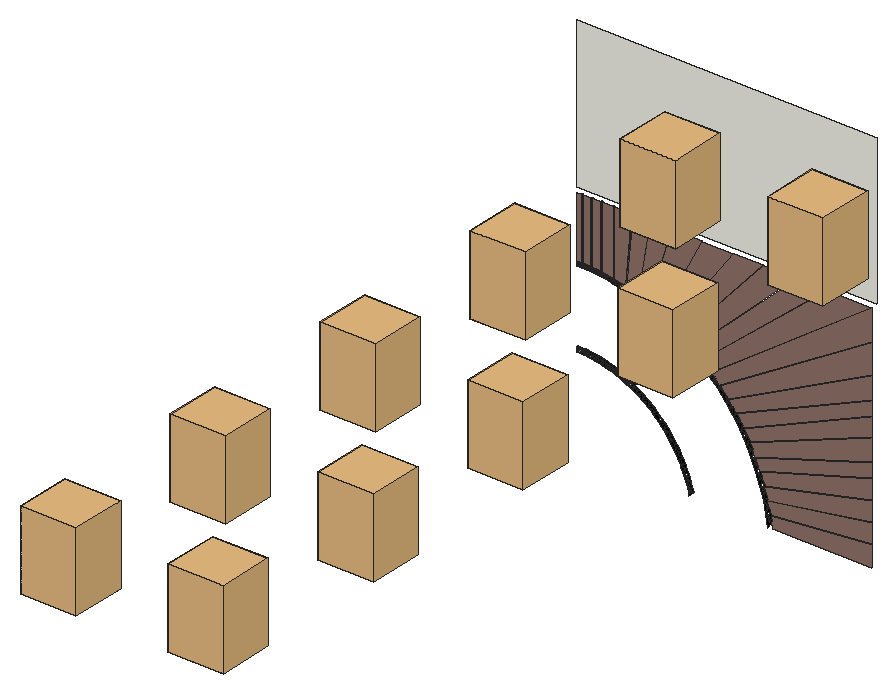
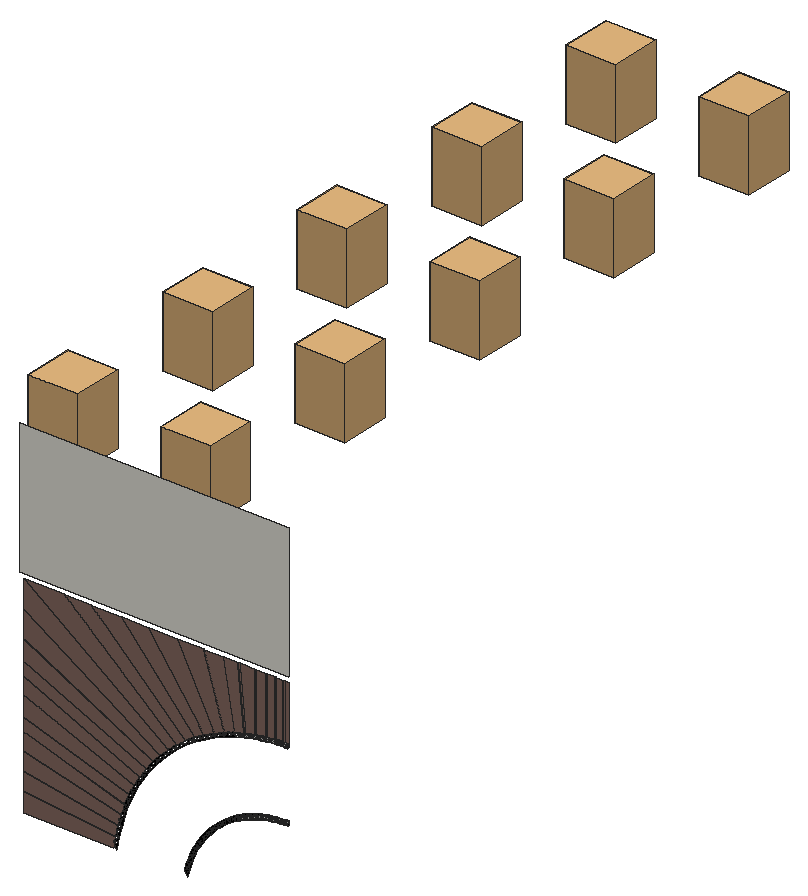
# SketchUp Ruby script. Lengths in inches.
U = 1.inch
M = Sketchup.active_model
def pt(a) = Geom::Point3d.new(a.map { |v| v * U })
def face(e, loops, mat)
  f = e.add_face(loops[0].map { |a| pt(a) })
  loops[1..].each { |l| e.add_face(l.map { |a| pt(a) }).erase! }
  f.material = f.back_material = mat if mat
  f
end
# faces: each face lists its corners as indices into pts; further lists are holes
def faces(e, pts, list, mat = nil) = list.each { |f| face(e, (f[0].is_a?(Array) ? f : [f]).map { |l| l.map { |i| pts[i] } }, mat) }
# xy, xz, yz: faces in a plane at the given z, y or x. An outline is a flat list of corners, or four numbers for a rectangle; further outlines are holes
def ring(l) = l.size == 4 ? [[l[0], l[1]], [l[2], l[1]], [l[2], l[3]], [l[0], l[3]]] : l.each_slice(2).to_a
def flat(e, list, mat, &to3) = list.each { |f| face(e, (f[0].is_a?(Array) ? f : [f]).map { |l| ring(l).map { |u, v| to3.(u, v) } }, mat) }
def xy(e, z, list, mat = nil) = flat(e, list, mat) { |x, y| [x, y, z] }
def xz(e, y, list, mat = nil) = flat(e, list, mat) { |x, z| [x, y, z] }
def yz(e, x, list, mat = nil) = flat(e, list, mat) { |y, z| [x, y, z] }
def lines(e, pts, list) = list.each { |a, b| e.add_line(pt(pts[a]), pt(pts[b])) }
# prism: a flat outline (further loops are holes) pulled along v
def prism(e, loops, v, mat = nil)
  f = face(e, loops, mat); d = Geom::Vector3d.new(v.map { |x| x * U })
  f.pushpull(f.normal.samedirection?(d) ? d.length : -d.length)
end
def box(e, o, s, mat = nil) = prism(e, [[o, [o[0] + s[0], o[1], o[2]], [o[0] + s[0], o[1] + s[1], o[2]], [o[0], o[1] + s[1], o[2]]]], [0, 0, s[2]], mat)
def at(x, y, z, deg = 0) = Geom::Transformation.translation(pt([x, y, z])) * Geom::Transformation.rotation(ORIGIN, Z_AXIS, deg.degrees)
def axes(o, x, y, z) = Geom::Transformation.new([*x, 0, *y, 0, *z, 0, *pt(o).to_a, 1])
def part(name) = M.definitions.add(name)
# library, detail: a bought-in or finely detailed component or shape, given as its bounding box
def library(name, o, s) = part(name).tap { |d| box(d.entities, o, s) }
def detail(e, o, s) = box(e.add_group.entities, o, s)
def put(e, d, t, mat = nil) = e.add_instance(d, t).tap { |i| i.material = mat if mat }
def group(e, t, mat = nil) = e.add_group.tap { |g| g.transformation = t; g.material = mat if mat }.entities
root = M.entities
M.materials.add("Tafisa-Gardenia-or-Gardenia-PM775-4K").color = [246, 245, 235]
M.materials.add("Tafisa-Terrarossa-PM780-4K").color = [148, 117, 107]
M.materials.add("Uniboard-L19-Putty-4K").color = [187, 181, 160]
M.materials.add("[Color M09]").color = [0, 0, 0]
c1 = library("Group\#8",[0,0,0],[8.9,8.9,12.62])
xy(root,78.776,[[101.221,138,101.236,138.157]],"Uniboard-L19-Putty-4K")
xy(root,79.385,[[100.715,138,100.814,138.157],[101.129,138,101.325,138.157]])
xy(root,89.291,[[101.327,138,101.445,138.157],[102.829,138,102.947,138.157],[104.449,138,104.567,138.157],[106.403,138,106.521,138.157],[109.35,138,109.469,138.157]])
xz(root,138,[[100.618,90.118,148.5,114]],"Tafisa-Gardenia-or-Gardenia-PM775-4K")
xz(root,138,[[131.874,51.949,147.791,51.949,147.791,55.307,131.583,53.786,131.719,52.926],[131.564,53.903,147.791,55.426,147.791,58.431,131.159,55.719,131.349,54.869],[131.133,55.835,147.791,58.551,147.791,61.594,130.614,57.622,130.857,56.785],[130.581,57.735,147.791,61.716,147.791,64.758,129.95,59.486,130.245,58.666],[129.91,59.598,147.791,64.881,147.791,67.121,129.171,61.305,129.517,60.506],
  [129.124,61.414,147.791,67.244,147.791,70.662,128.279,63.072,128.675,62.296],[128.226,63.177,147.791,70.788,147.791,73.694,127.279,64.778,127.722,64.029],[127.218,64.881,147.791,73.823,147.791,75.943,126.106,66.518,126.662,65.699],[126.031,66.614,126.059,66.626,147.744,76.051,147.791,76.072,147.791,79.556,124.893,68.082,125.499,67.3],[124.812,68.173,124.84,68.187,147.738,79.662,147.791,79.689,147.791,84.298,123.584,69.566,124.238,68.824],
  [123.498,69.652,123.522,69.667,147.73,84.398,147.791,84.436,147.791,89.291,122.184,70.966],[122.093,71.046,122.116,71.062,147.588,89.291,140.748,89.291,120.7,72.275,121.442,71.62],[120.604,72.349,120.623,72.365,140.566,89.291,135.862,89.291,119.136,73.488,119.875,72.914],[119.036,73.556,119.055,73.573,135.69,89.291,130.503,89.291,117.499,74.6,118.38,74.001],[117.395,74.661,117.411,74.678,130.345,89.291,125.683,89.291,115.795,75.607,116.846,74.986],
  [115.689,75.662,115.7,75.677,125.537,89.291,120.629,89.291,114.032,76.506,114.914,76.057],[113.925,76.552,113.936,76.575,120.497,89.291,115.795,89.291,112.216,77.292,113.124,76.899],[112.106,77.331,112.111,77.346,115.674,89.291,112.335,89.291,112.332,89.272,110.47,77.943,110.467,77.922,111.285,77.627],[110.353,77.962,112.216,89.291,109.469,89.291,108.453,78.515,109.263,78.279],[108.337,78.541,109.35,89.291,106.521,89.291,106.521,78.946,107.566,78.713],
  [106.403,78.965,106.403,89.291,104.567,89.291,104.567,79.256,105.082,79.174,106.182,79],[104.449,79.267,104.449,89.291,102.947,89.291,102.947,79.409,103.996,79.31],[102.829,79.42,102.829,89.291,101.445,89.291,101.445,79.478,101.962,79.462,102.596,79.442],[100.618,79.482,101.327,89.291]],"Tafisa-Terrarossa-PM780-4K")
xz(root,138,[[[131.171,51.86,131.719,52.926,130.868,53.77],[131.234,52.254,131.05,53.415,131.567,52.902]],[[118.55,52.008,119.203,52.772,118.263,53.126,118.424,52.572],[118.617,52.275,118.543,52.602,118.45,52.924,118.995,52.719]],[[119.203,52.772,118.867,53.929,118.761,54.223,118.263,53.126],[119.016,52.974,118.429,53.195,118.748,53.897,118.749,53.891]],[[131.719,52.926,131.583,53.786,131.564,53.903,131.349,54.869,130.868,53.77],[131.537,53.282,131.016,53.799,131.31,54.471,131.442,53.88]],[[118.263,53.126,118.761,54.223,117.711,54.767,118.102,53.681],[118.288,53.48,118.219,53.719,117.933,54.514,118.6,54.168]],
  [[130.868,53.77,131.349,54.869,130.446,55.658],[130.906,54.168,130.65,55.315,131.198,54.835]],[[118.761,54.223,118.458,55.063,118.188,55.688,117.711,54.767],[118.539,54.477,117.877,54.82,118.178,55.401,118.344,55.018]],[[117.711,54.767,118.188,55.688,117.142,56.044,117.252,55.827],[117.721,55.054,117.384,55.831,118.013,55.618]],[[131.349,54.869,131.159,55.719,131.133,55.835,130.857,56.785,130.446,55.658],[131.144,55.213,130.592,55.696,130.843,56.386,131.012,55.804]],[[130.446,55.658,130.857,56.785,129.906,57.516],[130.459,56.058,130.132,57.186,130.709,56.742]],
  [[118.188,55.688,117.979,56.17,117.503,57.105,117.142,56.044],[117.965,55.894,117.298,56.121,117.526,56.79,117.868,56.117]],[[117.142,56.044,117.503,57.105,116.434,57.353,116.728,56.856],[117.119,56.359,116.836,56.916,116.686,57.168,117.343,57.016]],[[130.857,56.785,130.614,57.622,130.581,57.735,130.245,58.666,129.906,57.516],[130.631,57.115,130.049,57.563,130.257,58.267,130.462,57.697]],[[117.503,57.105,117.432,57.244,116.819,58.281,116.434,57.353],[117.264,57.287,116.603,57.44,116.838,58.007]],[[116.434,57.353,116.819,58.281,115.815,58.328,116.14,57.85],[116.415,57.628,116.244,57.916,116.055,58.194,116.638,58.166]],
  [[129.906,57.516,130.245,58.666,129.251,59.337],[129.894,57.916,129.496,59.021,130.1,58.614]],[[116.819,58.281,116.141,59.278,115.402,60.231,114.605,61.135,114.401,60.151,115.402,60.151,115.137,59.262,116.141,59.262,115.815,58.328],[114.581,60.298,114.689,60.819,115.148,60.298],[116.533,58.441,116.018,58.465,116.187,58.95],[115.333,59.408,115.478,59.894,115.855,59.408]],[[115.815,58.328,116.141,59.262,115.137,59.262,115.491,58.806],[115.788,58.534,115.566,58.861,115.327,59.169,116.01,59.169]],[[130.245,58.666,129.95,59.486,129.91,59.598,129.517,60.506,129.251,59.337],[130,58.982,129.391,59.392,129.554,60.108,129.795,59.552]],[[115.137,59.262,115.402,60.151,114.401,60.151,114.783,59.718],[115.099,59.463,114.855,59.778,114.608,60.058,115.277,60.058]],
  [[129.251,59.337,129.517,60.506,128.483,61.112],[129.214,59.734,128.747,60.813,129.376,60.445]],[[114.401,60.151,114.605,61.135,113.611,60.993,114.019,60.585],[114.348,60.353,114.087,60.648,113.809,60.927,114.487,61.024]],[[129.517,60.506,129.171,61.305,129.124,61.414,128.675,62.296,128.483,61.112],[129.252,60.805,128.619,61.176,128.737,61.901,129.012,61.361]],[[113.611,60.993,113.753,61.987,112.769,61.783,113.203,61.401],[113.518,61.271,113.293,61.497,113.053,61.708,113.596,61.821]],[[113.611,60.993,114.605,61.135,113.753,61.987],[113.721,61.103,113.819,61.789,114.407,61.201]],
  [[128.483,61.112,128.675,62.296,127.604,62.836],[128.421,61.507,127.887,62.554,128.538,62.226]],[[112.769,61.783,112.849,62.784,111.88,62.519,112.336,62.165],[112.659,62.055,112.42,62.266,112.168,62.462,112.703,62.608]],[[112.769,61.783,113.753,61.987,112.849,62.784],[112.914,61.947,112.959,62.512,113.469,62.062]],[[128.675,62.296,128.279,63.072,128.226,63.177,127.722,64.029,127.604,62.836],[128.392,62.578,127.736,62.908,127.808,63.639,128.117,63.117]],[[111.88,62.519,111.896,63.523,110.946,63.197,111.424,62.873],[111.753,62.783,111.501,62.979,111.237,63.158,111.762,63.338]],
  [[111.88,62.519,112.849,62.784,111.896,63.523],[112.014,62.692,112.023,63.258,112.561,62.841]],[[127.604,62.836,127.722,64.029,126.619,64.501],[127.518,63.226,126.92,64.237,127.589,63.951]],[[110.946,63.197,110.899,64.201,109.972,63.816,110.469,63.522],[110.803,63.453,110.539,63.633,110.264,63.795,110.777,64.008]],[[110.946,63.197,111.896,63.523,110.899,64.201],[111.069,63.378,111.043,63.944,111.605,63.562]],[[109.972,63.816,109.862,64.814,108.96,64.372,109.475,64.11],[109.869,63.974,109.515,64.184,109.149,64.37,109.791,64.686]],
  [[109.972,63.816,110.899,64.201,109.862,64.814],[110.083,64.004,110.021,64.567,110.606,64.221]],[[127.722,64.029,127.279,64.778,127.218,64.881,126.662,65.699,126.619,64.501],[127.422,64.293,126.747,64.582,126.773,65.315,127.113,64.814]],[[108.96,64.372,108.788,65.361,107.916,64.863,108.446,64.634],[108.848,64.524,108.481,64.71,108.104,64.874,108.725,65.229]],[[108.96,64.372,109.862,64.814,108.788,65.361],[109.024,64.497,108.9,65.21,109.673,64.816]],[[126.619,64.501,126.662,65.699,125.532,66.101],[126.509,64.885,125.848,65.857,126.535,65.613]],
  [[107.916,64.863,107.682,65.84,106.842,65.288,107.386,65.093],[107.794,65.008,107.417,65.171,107.03,65.311,107.627,65.704]],[[107.916,64.863,108.788,65.361,107.682,65.84],[107.971,64.992,107.803,65.696,108.6,65.351]],[[106.842,65.288,106.547,66.248,105.744,65.645,106.299,65.484],[106.622,65.52,106.343,65.62,106.059,65.703,106.47,66.012]],[[106.842,65.288,107.682,65.84,106.547,66.248],[106.923,65.513,106.768,66.017,107.364,65.802]],[[105.744,65.645,105.39,66.585,104.626,65.932,105.19,65.806],[105.51,65.862,105.226,65.945,104.937,66.009,105.328,66.344]],
  [[105.744,65.645,106.547,66.248,105.39,66.585],[105.811,65.874,105.625,66.368,106.233,66.191]],[[126.662,65.699,126.106,66.518,126.031,66.614,125.499,67.3,125.532,66.101],[126.346,65.944,125.654,66.19,125.634,66.923,126.005,66.445]],[[104.626,65.932,104.213,66.848,103.493,66.148,104.063,66.058],[104.378,66.134,104.09,66.199,103.797,66.245,104.167,66.603]],[[104.626,65.932,105.39,66.585,104.213,66.848],[104.678,66.165,104.461,66.646,105.079,66.508]],[[125.532,66.101,125.499,67.3,124.346,67.63],[125.397,66.477,124.677,67.406,125.377,67.205]],
  [[103.493,66.148,103.023,67.036,102.347,66.293,102.922,66.239],[103.232,66.334,102.94,66.381,102.646,66.409,102.992,66.789]],[[103.493,66.148,104.213,66.848,103.023,67.036],[103.53,66.384,103.283,66.85,103.909,66.751]],[[102.347,66.293,101.823,67.15,101.597,66.353,101.772,66.347],[102.076,66.462,101.784,66.49,101.871,66.796]],[[102.347,66.293,103.023,67.036,101.823,67.15],[102.37,66.53,102.094,66.98,102.725,66.921]],[[101.597,66.353,101.221,67.169,100.618,66.384,101.422,66.358],[101.37,66.503,100.901,66.518,101.19,66.894]],
  [[101.597,66.353,101.823,67.15,101.221,67.169],[101.565,66.764,101.447,67.018,101.635,67.012]],[[100.618,66.384,101.221,67.169,100.618,67.1875],[100.761,66.805,100.761,67.04,100.937,67.034]],[[125.499,67.3,124.893,68.082,124.812,68.173,124.238,68.824,124.346,67.63],[125.168,67.524,124.462,67.726,124.396,68.457,124.797,68.002]],[[124.346,67.63,124.238,68.824,123.067,69.081],[124.188,67.997,123.411,68.878,124.123,68.722]],[[124.238,68.824,123.584,69.566,122.884,70.266,123.067,69.081],[123.894,69.027,123.177,69.184,123.065,69.91,123.493,69.481]],
  [[123.067,69.081,122.884,70.266,121.699,70.449],[122.886,69.4375,122.055,70.268,122.775,70.157]],[[122.884,70.266,122.184,70.966,122.093,71.046,121.442,71.62,121.699,70.449],[122.528,70.447,121.802,70.559,121.645,71.276,122.099,70.875]],[[121.699,70.449,121.442,71.62,120.248,71.728],[121.496,70.793,120.615,71.57,121.34,71.505]],[[121.442,71.62,120.7,72.275,120.604,72.349,119.875,72.914,120.248,71.728],[121.157,71.743,120.321,71.819,120.06,72.648,120.638,72.2]],[[120.248,71.728,119.875,72.914,118.719,72.914],[120.063,71.994,119.001,72.817,119.804,72.817]],
  [[118.719,72.914,118.38,74.001,117.119,74.001],[118.544,73.149,117.433,73.905,118.309,73.905]],[[118.719,72.914,119.875,72.914,119.136,73.488,119.036,73.556,118.38,74.001],[118.79,73.011,118.555,73.766,119.079,73.409,119.593,73.011]],[[117.119,74.001,116.846,74.986,115.454,74.986],[116.962,74.207,115.807,74.89,116.773,74.89]],[[117.119,74.001,118.38,74.001,117.499,74.6,117.395,74.661,116.846,74.986],[117.193,74.098,117.003,74.781,117.447,74.518,118.066,74.098]],[[115.454,74.986,114.914,76.057,113.73,75.864],[115.235,75.206,114.037,75.816,114.859,75.95]],
  [[115.454,74.986,116.846,74.986,115.795,75.607,115.689,75.662,114.914,76.057],[115.513,75.083,115.133,75.837,115.749,75.523,116.493,75.083]],[[113.73,75.864,113.124,76.899,111.955,76.633],[113.497,76.07,112.264,76.604,113.076,76.789]],[[113.73,75.864,114.914,76.057,114.032,76.506,113.925,76.552,113.124,76.899],[113.78,75.97,113.356,76.693,113.991,76.419,114.607,76.105]],[[111.955,76.633,111.285,77.627,109.87,77.365,110.134,77.288],[111.709,76.824,110.272,77.341,111.24,77.521]],[[111.955,76.633,113.124,76.899,112.216,77.292,112.106,77.331,111.285,77.627],[111.998,76.742,111.53,77.436,112.18,77.202,112.814,76.928]],
  [[109.87,77.365,109.263,78.279,108.277,77.828],[109.643,77.531,108.553,77.848,109.228,78.157]],[[109.87,77.365,111.285,77.627,110.467,77.922,110.353,77.962,109.263,78.279],[109.915,77.472,109.489,78.113,110.324,77.871,110.916,77.657]],[[108.277,77.828,107.566,78.713,106.612,78.2],[108.029,77.982,106.886,78.238,107.541,78.59]],[[108.277,77.828,109.263,78.279,108.453,78.515,108.337,78.541,107.566,78.713],[108.305,77.947,107.814,78.558,108.429,78.421,108.986,78.259]],[[106.612,78.2,106.182,79,105.433,78.401,106.389,78.25],[106.427,78.34,106.407,78.345,105.664,78.462,106.151,78.852]],
  [[106.612,78.2,107.566,78.713,106.521,78.946,106.403,78.965,106.182,79],[106.651,78.331,106.359,78.874,106.503,78.851,107.292,78.675]],[[105.433,78.401,105.082,79.174,104.478,78.553],[105.271,78.525,104.677,78.619,105.052,79.006]],[[105.433,78.401,106.182,79,105.082,79.174],[105.47,78.554,105.244,79.051,105.951,78.939]],[[104.478,78.553,103.996,79.31,103.515,78.644],[104.29,78.667,103.692,78.724,103.991,79.138]],[[104.478,78.553,105.082,79.174,104.567,79.256,104.449,79.267,103.996,79.31],[104.494,78.708,104.184,79.195,104.555,79.16,104.883,79.108]],
  [[103.515,78.644,102.947,79.409,102.552,78.735],[103.308,78.76,102.712,78.817,102.956,79.234]],[[103.515,78.644,103.996,79.31,102.947,79.409],[103.514,78.807,103.154,79.292,103.819,79.23]],[[102.552,78.735,101.962,79.462,101.327,78.773],[102.344,78.838,101.541,78.863,101.957,79.315]],[[102.552,78.735,102.947,79.409,102.829,79.42,102.596,79.442,101.962,79.462],[102.539,78.904,102.17,79.359,102.59,79.346,102.787,79.327]],[[101.327,78.773,100.972,79.482,100.618,78.795,101.221,78.776,101.221,78.875,101.236,78.776],[101.168,78.875,100.774,78.887,100.971,79.269]],
  [[101.327,78.773,101.962,79.462,101.445,79.478,101.327,79.482,100.972,79.482],[101.351,78.942,101.129,79.385,101.325,79.385,101.747,79.372]],[101.221,78.776,101.236,78.776,101.221,78.875],[[100.618,78.795,100.972,79.482,100.618,79.482],[100.715,79.193,100.715,79.385,100.814,79.385]]],"[Color M09]")
yz(root,100.715,[[138,79.193,138.157,79.385]])
yz(root,100.761,[[138,66.805,138.157,67.04]])
yz(root,101.327,[[138,79.482,138.157,89.291]],"Tafisa-Terrarossa-PM780-4K")
yz(root,101.445,[[138,79.478,138.157,79.482]])
yz(root,101.445,[[138,79.482,138.157,89.291]],"Tafisa-Terrarossa-PM780-4K")
yz(root,102.829,[[138,79.42,138.157,89.291]],"Tafisa-Terrarossa-PM780-4K")
yz(root,102.947,[[138,79.409,138.157,89.291]],"Tafisa-Terrarossa-PM780-4K")
yz(root,104.449,[[138,79.267,138.157,89.291]],"Tafisa-Terrarossa-PM780-4K")
yz(root,104.567,[[138,79.256,138.157,89.291]],"Tafisa-Terrarossa-PM780-4K")
yz(root,106.403,[[138,78.965,138.157,89.291]],"Tafisa-Terrarossa-PM780-4K")
yz(root,106.521,[[138,78.946,138.157,89.291]],"Tafisa-Terrarossa-PM780-4K")
p = [[109.475,138,64.11],[108.96,138,64.372],[108.96,138.157,64.372],[109.475,138.157,64.11],[109.149,138,64.37],[109.515,138,64.184],
  [109.515,138.157,64.184],[109.149,138.157,64.37],[108.446,138,64.634],[108.446,138.157,64.634],[108.481,138,64.71],[108.848,138,64.524],
  [108.848,138.157,64.524],[108.481,138.157,64.71],[108.725,138,65.229],[108.725,138.157,65.229],[108.9,138,65.21],[109.024,138,64.497],
  [109.024,138.157,64.497],[108.9,138.157,65.21],[109.673,138,64.816],[109.673,138.157,64.816],[107.916,138,64.863],[107.916,138.157,64.863],
  [108.104,138,64.874],[108.104,138.157,64.874],[108.788,138,65.361],[109.862,138,64.814],[109.862,138.157,64.814],[108.788,138.157,65.361],
  [107.386,138,65.093],[107.386,138.157,65.093],[107.417,138,65.171],[107.794,138,65.008],[107.794,138.157,65.008],[107.417,138.157,65.171],
  [107.627,138,65.704],[107.627,138.157,65.704],[107.803,138,65.696],[107.971,138,64.992],[107.971,138.157,64.992],[107.803,138.157,65.696],
  [108.6,138,65.351],[108.6,138.157,65.351],[106.842,138,65.288],[106.842,138.157,65.288],[107.03,138,65.311],[107.03,138.157,65.311],
  [106.299,138,65.484],[106.299,138.157,65.484],[107.682,138,65.84],[107.682,138.157,65.84],[105.744,138,65.645],[105.744,138.157,65.645],
  [106.343,138,65.62],[106.622,138,65.52],[106.622,138.157,65.52],[106.343,138.157,65.62],[106.47,138,66.012],[106.47,138.157,66.012],
  [106.768,138,66.017],[106.923,138,65.513],[106.923,138.157,65.513],[106.768,138.157,66.017],[107.364,138,65.802],[107.364,138.157,65.802],
  [105.19,138,65.806],[105.19,138.157,65.806],[106.059,138,65.703],[106.059,138.157,65.703],[104.626,138,65.932],[104.626,138.157,65.932],
  [106.547,138,66.248],[106.547,138.157,66.248],[104.063,138,66.058],[104.063,138.157,66.058],[104.937,138,66.009],[105.226,138,65.945],
  [105.226,138.157,65.945],[104.937,138.157,66.009],[105.51,138,65.862],[105.51,138.157,65.862],[105.328,138,66.344],[105.328,138.157,66.344],
  [105.625,138,66.368],[105.811,138,65.874],[105.811,138.157,65.874],[105.625,138.157,66.368],[106.233,138,66.191],[106.233,138.157,66.191],
  [103.493,138,66.148],[102.922,138,66.239],[102.922,138.157,66.239],[103.493,138.157,66.148],[104.09,138,66.199],[104.378,138,66.134],
  [104.378,138.157,66.134],[104.09,138.157,66.199],[104.167,138,66.603],[104.167,138.157,66.603],[102.347,138,66.293],[102.347,138.157,66.293],
  [103.797,138,66.245],[103.797,138.157,66.245],[104.461,138,66.646],[104.678,138,66.165],[104.678,138.157,66.165],[104.461,138.157,66.646],
  [105.079,138,66.508],[105.079,138.157,66.508],[105.39,138,66.585],[105.39,138.157,66.585],[101.772,138,66.347],[101.597,138,66.353],
  [101.597,138.157,66.353],[101.772,138.157,66.347],[102.94,138,66.381],[103.232,138,66.334],[103.232,138.157,66.334],[102.94,138.157,66.381],
  [102.992,138,66.789],[102.992,138.157,66.789],[101.422,138,66.358],[100.618,138,66.384],[100.618,138.157,66.384],[101.422,138.157,66.358],
  [102.646,138,66.409],[102.646,138.157,66.409],[103.283,138,66.85],[103.53,138,66.384],[103.53,138.157,66.384],[103.283,138.157,66.85],
  [103.909,138,66.751],[103.909,138.157,66.751],[101.19,138,66.894],[100.901,138,66.518],[100.901,138.157,66.518],[101.19,138.157,66.894],
  [101.37,138,66.503],[101.37,138.157,66.503],[101.871,138,66.796],[101.784,138,66.49],[101.784,138.157,66.49],[101.871,138.157,66.796],
  [102.076,138,66.462],[102.076,138.157,66.462],[102.094,138,66.98],[102.37,138,66.53],[102.37,138.157,66.53],[102.094,138.157,66.98],
  [102.725,138,66.921],[102.725,138.157,66.921],[104.213,138,66.848],[104.213,138.157,66.848],[100.761,138,66.805],[100.937,138,67.034],
  [100.937,138.157,67.034],[100.761,138.157,66.805],[101.447,138,67.018],[101.565,138,66.764],[101.565,138.157,66.764],[101.447,138.157,67.018],
  [101.635,138,67.012],[101.635,138.157,67.012],[103.023,138,67.036],[103.023,138.157,67.036],[100.761,138,67.04],[100.761,138.157,67.04],
  [101.823,138,67.15],[101.823,138.157,67.15],[101.221,138,67.169],[101.221,138.157,67.169],[100.618,138,67.1875],[100.618,138.157,67.1875],
  [109.87,138,77.365],[108.277,138,77.828],[108.277,138.157,77.828],[109.87,138.157,77.365],[108.553,138,77.848],[109.643,138,77.531],
  [109.643,138.157,77.531],[108.553,138.157,77.848],[106.612,138,78.2],[106.612,138.157,78.2],[109.228,138,78.157],[109.228,138.157,78.157],
  [107.814,138,78.558],[108.305,138,77.947],[108.305,138.157,77.947],[107.814,138.157,78.558],[108.986,138,78.259],[108.986,138.157,78.259],
  [106.886,138,78.238],[108.029,138,77.982],[108.029,138.157,77.982],[106.886,138.157,78.238],[107.541,138,78.59],[107.541,138.157,78.59],
  [106.389,138,78.25],[105.433,138,78.401],[105.433,138.157,78.401],[106.389,138.157,78.25],[105.664,138,78.462],[106.407,138,78.345],
  [106.407,138.157,78.345],[105.664,138.157,78.462],[106.427,138,78.34],[106.151,138,78.852],[106.151,138.157,78.852],[106.427,138.157,78.34],
  [106.359,138,78.874],[106.651,138,78.331],[106.651,138.157,78.331],[106.359,138.157,78.874],[107.292,138,78.675],[107.292,138.157,78.675],
  [108.429,138,78.421],[108.429,138.157,78.421],[104.478,138,78.553],[104.478,138.157,78.553],[104.677,138,78.619],[105.271,138,78.525],
  [105.271,138.157,78.525],[104.677,138.157,78.619],[105.052,138,79.006],[105.052,138.157,79.006],[108.337,138,78.541],[108.453,138,78.515],
  [108.453,138.157,78.515],[108.337,138.157,78.541],[109.35,138,89.291],[109.35,138.157,89.291],[109.469,138,89.291],[109.469,138.157,89.291],
  [103.515,138,78.644],[102.552,138,78.735],[102.552,138.157,78.735],[103.515,138.157,78.644],[105.244,138,79.051],[105.47,138,78.554],
  [105.47,138.157,78.554],[105.244,138.157,79.051],[105.951,138,78.939],[105.951,138.157,78.939],[101.327,138,78.773],[101.327,138.157,78.773],
  [103.991,138,79.138],[103.692,138,78.724],[103.692,138.157,78.724],[103.991,138.157,79.138],[104.29,138,78.667],[104.29,138.157,78.667],
  [104.184,138,79.195],[104.494,138,78.708],[104.494,138.157,78.708],[104.184,138.157,79.195],[104.883,138,79.108],[104.883,138.157,79.108],
  [106.503,138,78.851],[106.503,138.157,78.851],[101.221,138,78.776],[100.618,138,78.795],[100.618,138.157,78.795],[101.221,138.157,78.776],
  [101.236,138,78.776],[101.236,138.157,78.776],[101.541,138,78.863],[102.344,138,78.838],[102.344,138.157,78.838],[101.541,138.157,78.863],
  [101.957,138,79.315],[101.957,138.157,79.315],[102.956,138,79.234],[102.712,138,78.817],[102.712,138.157,78.817],[102.956,138.157,79.234],
  [103.308,138,78.76],[103.308,138.157,78.76],[103.154,138,79.292],[103.514,138,78.807],[103.514,138.157,78.807],[103.154,138.157,79.292],
  [103.819,138,79.23],[103.819,138.157,79.23],[100.971,138,79.269],[100.774,138,78.887],[100.774,138.157,78.887],[100.971,138.157,79.269],
  [101.168,138,78.875],[101.168,138.157,78.875],[101.129,138,79.385],[101.351,138,78.942],[101.351,138.157,78.942],[101.129,138.157,79.385],
  [101.747,138,79.372],[101.747,138.157,79.372],[102.17,138,79.359],[102.539,138,78.904],[102.539,138.157,78.904],[102.17,138.157,79.359],
  [102.787,138,79.327],[102.787,138.157,79.327],[106.403,138,78.965],[106.521,138,78.946],[106.521,138.157,78.946],[106.403,138.157,78.965],
  [104.555,138,79.16],[104.555,138.157,79.16],[100.715,138,79.193],[100.814,138,79.385],[100.814,138.157,79.385],[100.715,138.157,79.193],
  [102.59,138,79.346],[102.59,138.157,79.346],[104.449,138,79.267],[104.567,138,79.256],[104.567,138.157,79.256],[104.449,138.157,79.267],
  [101.325,138,79.385],[101.325,138.157,79.385],[102.829,138,79.42],[102.947,138,79.409],[102.947,138.157,79.409],[102.829,138.157,79.42],
  [101.327,138,79.482],[101.445,138,79.478],[101.445,138.157,79.478],[101.327,138.157,79.482],[125.537,138,89.291],[125.587,138,89.361],
  [130.345,138,89.291],[130.414,138,89.37],[135.69,138,89.291],[135.781,138,89.377],[140.566,138,89.291],[140.672,138,89.381],
  [147.723,138,89.387],[147.588,138,89.291],[127.265,138,64.773],[127.279,138,64.778],[147.791,138,73.694],[147.838,138,73.714],
  [128.268,138,63.067],[128.279,138,63.072],[147.791,138,70.662],[147.834,138,70.678],[129.159,138,61.301],[129.171,138,61.305],
  [147.791,138,67.121],[147.827,138,67.132],[129.944,138,59.484],[129.95,138,59.486],[147.791,138,64.758],[147.825,138,64.768],
  [130.607,138,57.62],[130.614,138,57.622],[147.791,138,61.594],[147.818,138,61.601],[131.152,138,55.718],[131.159,138,55.719],
  [147.791,138,58.431],[147.81,138,58.434],[131.575,138,53.786],[131.583,138,53.786],[147.791,138,55.307],[147.802,138,55.308],
  [131.874,138,51.83],[131.885,138,51.83],[120.497,138,89.291],[120.533,138,89.361],[115.674,138,89.291],[115.69,138,89.345],
  [108.335,138,78.526],[109.352,138,89.302],[106.403,138,78.946],[104.449,138,79.256],[102.829,138,79.409]]
faces(root,p,[[0,1,2,3],[1,8,9,2],[8,22,23,9],[26,27,28,29],[22,30,31,23],[30,44,45,31],[44,48,49,45],[50,26,29,51],
  [48,52,53,49],[52,66,67,53],[66,70,71,67],[72,50,51,73],[70,74,75,71],[90,91,92,93],[74,90,93,75],[91,100,101,92],
  [110,72,73,111],[112,113,114,115],[100,112,115,101],[122,123,124,125],[113,122,125,114],[152,110,111,153],[164,152,153,165],[168,164,165,169],
  [170,168,169,171],[172,170,171,173]],"[Color M09]")
faces(root,p,[[4,5,6,7],[10,11,12,13],[11,14,15,12],[16,17,18,19],[17,20,21,18],[24,10,13,25],[20,16,19,21],[14,24,25,15],
  [32,33,34,35],[33,36,37,34],[38,39,40,41],[39,42,43,40],[46,32,35,47],[36,46,47,37],[42,38,41,43],[54,55,56,57],
  [55,58,59,56],[60,61,62,63],[61,64,65,62],[68,54,57,69],[58,68,69,59],[64,60,63,65],[76,77,78,79],[77,80,81,78],
  [80,82,83,81],[84,85,86,87],[85,88,89,86],[82,76,79,83],[94,95,96,97],[95,98,99,96],[102,94,97,103],[98,102,103,99],
  [104,105,106,107],[105,108,109,106],[88,84,87,89],[116,117,118,119],[117,120,121,118],[126,116,119,127],[120,126,127,121],[128,129,130,131],
  [129,132,133,130],[134,135,136,137],[135,138,139,136],[138,134,137,139],[140,141,142,143],[141,144,145,142],[144,140,143,145],[146,147,148,149],
  [147,150,151,148],[108,104,107,109],[154,155,156,157],[158,159,160,161],[159,162,163,160],[132,128,131,133],[150,146,149,151],[155,166,167,156],
  [162,158,161,163],[178,179,180,181],[184,178,181,185],[186,187,188,189],[187,190,191,188],[192,193,194,195],[193,196,197,194],[196,192,195,197],
  [202,203,204,205],[206,207,208,209],[203,206,209,204],[210,211,212,213],[211,214,215,212],[190,216,217,191],[216,186,189,217],[220,221,222,223],
  [221,224,225,222],[207,202,205,208],[226,227,228,229],[224,220,223,225],[238,239,240,241],[239,242,243,240],[246,247,248,249],[247,250,251,248],
  [250,246,249,251],[252,253,254,255],[253,256,257,254],[214,258,259,215],[266,267,268,269],[267,270,271,268],[272,273,274,275],[273,276,277,274],
  [276,272,275,277],[278,279,280,281],[279,282,283,280],[284,285,286,287],[285,288,289,286],[288,284,287,289],[290,291,292,293],[291,294,295,292],
  [270,266,269,271],[296,297,298,299],[297,300,301,298],[242,238,241,243],[258,210,213,259],[302,303,304,305],[256,306,307,257],[308,309,310,311],
  [282,278,281,283],[306,252,255,307],[312,296,299,313],[300,312,313,301],[314,315,316,317],[294,318,319,295],[320,321,322,323],[324,325,326,327]])
faces(root,p,[[174,175,176,177],[175,182,183,176],[198,199,200,201],[182,198,201,183],[199,218,219,200],[234,235,236,237],[218,234,237,219],[235,244,245,236],
  [260,261,262,263],[244,264,265,245]],"Uniboard-L19-Putty-4K")
faces(root,p,[[230,226,229,231],[227,232,233,228]],"Tafisa-Terrarossa-PM780-4K")
lines(root,p,[[328,329],[330,331],[332,333],[334,335],[336,337],[338,339],[340,341],[342,343],[344,345],[346,347],[348,349],[350,351],
  [352,353],[354,355],[356,357],[358,359],[360,361],[362,363],[364,365],[366,367],[368,369],[370,371],[372,226],[230,373],
  [374,302],[375,314],[320,376]])
put(root,c1,at(123.66,-2.26,101.38))
put(root,c1,at(147.28,-2.26,101.38))
put(root,c1,at(123.66,27.74,101.38))
put(root,c1,at(147.28,27.74,101.38))
put(root,c1,at(123.66,57.74,101.38))
put(root,c1,at(147.28,57.74,101.38))
put(root,c1,at(123.66,87.74,101.38))
put(root,c1,at(147.28,87.74,101.38))
put(root,c1,at(123.66,117.74,101.38))
put(root,c1,at(147.28,117.74,101.38))
